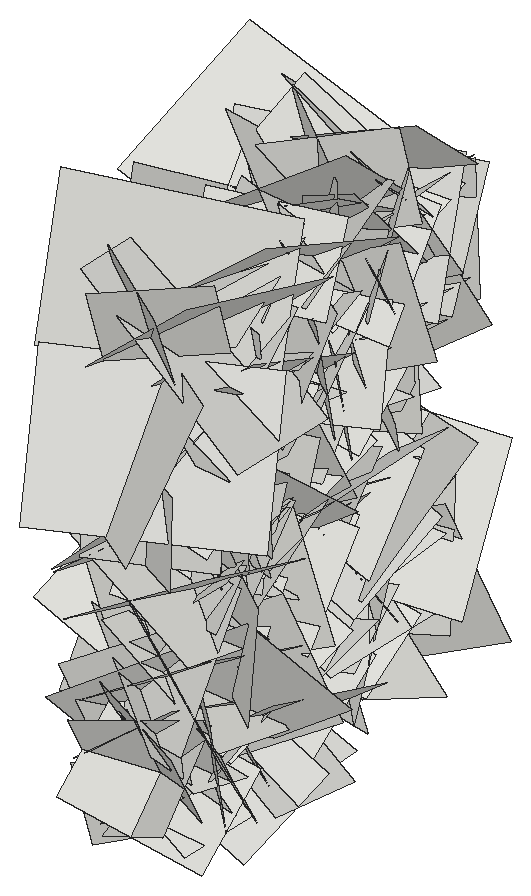
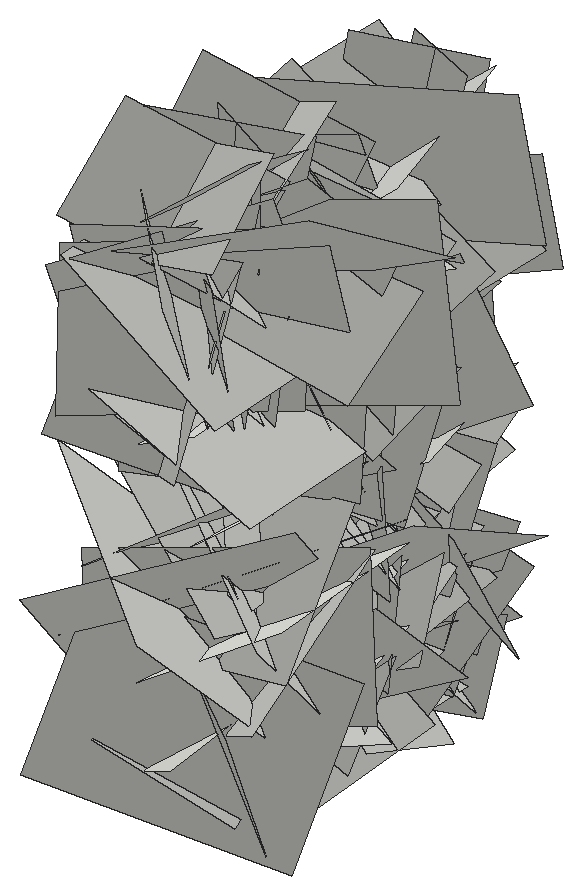
# SketchUp Ruby script. Lengths in inches.
U = 1.inch
M = Sketchup.active_model
def pt(a) = Geom::Point3d.new(a.map { |v| v * U })
def face(e, loops, mat)
  f = e.add_face(loops[0].map { |a| pt(a) })
  loops[1..].each { |l| e.add_face(l.map { |a| pt(a) }).erase! }
  f.material = f.back_material = mat if mat
  f
end
# faces: each face lists its corners as indices into pts; further lists are holes
def faces(e, pts, list, mat = nil) = list.each { |f| face(e, (f[0].is_a?(Array) ? f : [f]).map { |l| l.map { |i| pts[i] } }, mat) }
# xy, xz, yz: faces in a plane at the given z, y or x. An outline is a flat list of corners, or four numbers for a rectangle; further outlines are holes
def ring(l) = l.size == 4 ? [[l[0], l[1]], [l[2], l[1]], [l[2], l[3]], [l[0], l[3]]] : l.each_slice(2).to_a
def flat(e, list, mat, &to3) = list.each { |f| face(e, (f[0].is_a?(Array) ? f : [f]).map { |l| ring(l).map { |u, v| to3.(u, v) } }, mat) }
def xy(e, z, list, mat = nil) = flat(e, list, mat) { |x, y| [x, y, z] }
def xz(e, y, list, mat = nil) = flat(e, list, mat) { |x, z| [x, y, z] }
def yz(e, x, list, mat = nil) = flat(e, list, mat) { |y, z| [x, y, z] }
def lines(e, pts, list) = list.each { |a, b| e.add_line(pt(pts[a]), pt(pts[b])) }
# prism: a flat outline (further loops are holes) pulled along v
def prism(e, loops, v, mat = nil)
  f = face(e, loops, mat); d = Geom::Vector3d.new(v.map { |x| x * U })
  f.pushpull(f.normal.samedirection?(d) ? d.length : -d.length)
end
def box(e, o, s, mat = nil) = prism(e, [[o, [o[0] + s[0], o[1], o[2]], [o[0] + s[0], o[1] + s[1], o[2]], [o[0], o[1] + s[1], o[2]]]], [0, 0, s[2]], mat)
def at(x, y, z, deg = 0) = Geom::Transformation.translation(pt([x, y, z])) * Geom::Transformation.rotation(ORIGIN, Z_AXIS, deg.degrees)
def axes(o, x, y, z) = Geom::Transformation.new([*x, 0, *y, 0, *z, 0, *pt(o).to_a, 1])
def part(name) = M.definitions.add(name)
# library, detail: a bought-in or finely detailed component or shape, given as its bounding box
def library(name, o, s) = part(name).tap { |d| box(d.entities, o, s) }
def detail(e, o, s) = box(e.add_group.entities, o, s)
def put(e, d, t, mat = nil) = e.add_instance(d, t).tap { |i| i.material = mat if mat }
def group(e, t, mat = nil) = e.add_group.tap { |g| g.transformation = t; g.material = mat if mat }.entities
root = M.entities
c1 = part("Component\#6")
p = [[0.01,0,0],[0,3.24,4.54],[4.32,3.24,4.54],[4.33,0,0]]
faces(c1.entities,p,[[0,1,2,3]])
put(root,c1,axes([18.5,183.19,37.72],[-0.19709,-1.17807,-0.70591],[-0.26547,-0.67132,1.18631],[-1.43137,0.28672,-0.12282]))
put(root,c1,axes([18.5,179.625,37.91],[-0.28026,0.12179,-1.29213],[-0.26115,-1.29941,-0.07206],[-1.35072,0.22596,0.28204]))
put(root,c1,axes([18.5,177.28,39.83],[-0.04784,1.11638,-0.64936],[-0.22797,-0.64718,-1.09769],[-1.34988,0.06974,0.20839]))
put(root,c1,axes([18.5,183.77,26.5],[-0.0762,-1.33255,-0.21023],[-0.04546,-0.20817,1.33413],[-1.42926,0.07766,-0.03122]))
put(root,c1,axes([18.5,177.96,25.04],[-0.10915,-1.1796,-0.55067],[-0.03689,-0.5497,1.18402],[-1.37942,0.10803,0.01191]))
put(root,c1,axes([18.5,175.66,39.88],[0.03914,-0.32872,-1.22009],[-0.25418,-1.20026,0.31612],[-1.31508,0.2222,-0.09741]))
put(root,c1,axes([18.5,169.91,24.28],[0.0494,0.58776,1.07494],[-0.25393,1.05932,-0.56884],[-1.27358,-0.18841,0.15511]))
put(root,c1,axes([18.5,178.68,21.25],[-0.14964,-1.02559,0.91665],[0.24358,0.89093,1.03221],[-1.43757,0.25771,0.07948]))
put(root,c1,axes([18.5,178.09,32.9],[-0.18757,-0.47698,-1.21124],[0.23196,-1.21588,0.44684],[-1.36024,-0.14157,0.24323]))
put(root,c1,axes([18.5,178.49,34.59],[-0.00763,1.14917,-0.03145],[-0.21412,-0.03223,-1.13128],[-1.19962,-0.00155,0.20212]))
put(root,c1,axes([18.5,182.31,23.94],[0.04872,-1.30982,0.04089],[-0.01644,0.04037,1.31055],[-1.38898,-0.04642,-0.01408]))
put(root,c1,axes([18.5,174.06,31.875],[-0.08593,-0.00736,1.08266],[-0.18405,1.07173,-0.00571],[-1.1328,-0.17357,-0.0812]))
put(root,c1,axes([18.5,177.97,39.67],[0.02985,0.75948,-0.84861],[-0.27983,-0.8214,-0.74388],[-1.17429,0.21504,0.15569]))
put(root,c1,axes([18.5,180.07,24.39],[0.06666,-0.76105,0.92501],[-0.21989,0.90537,0.75899],[-1.25053,-0.19976,-0.08415]))
put(root,c1,axes([18.5,182.77,28.7],[0.0358,-0.11408,-1.31406],[0.04325,-1.31377,0.1151],[-1.39747,-0.04358,-0.0301]))
put(root,c1,axes([18.5,179.04,23.77],[-0.11323,-0.75693,-0.7774],[-0.09292,-0.77258,0.76428],[-1.14637,0.13739,0.01483]))
put(root,c1,axes([18.5,183.25,38.77],[0.07927,-0.40868,-1.12281],[-0.1988,-1.11508,0.39337],[-1.25087,0.15132,-0.13368]))
put(root,c1,axes([18.5,172.47,36.95],[-0.1233,0.89549,0.4145],[-0.21728,0.38634,-0.89217],[-1.02316,-0.18996,0.13951]))
put(root,c1,axes([18.5,175.96,26.52],[-0.03553,0.82214,0.9074],[0.07429,0.90754,-0.81968],[-1.2958,0.02948,-0.07187]))
put(root,c1,axes([18.5,182.25,27.43],[0.1955,0.46825,-1.21407],[-0.10064,-1.21809,-0.48422],[-1.37564,0.15566,-0.13711]))
put(root,c1,axes([18.5,180.75,35.09],[0.01445,0.08276,-1.11066],[-0.1396,-1.10283,-0.0838],[-1.17228,0.13235,-0.00371]))
put(root,c1,axes([14.53,172.58,29],[-0.14706,-0.68518,0.03236],[-0.10474,0.05263,0.69082],[0.71951,-0.13238,0.10718]))
put(root,c1,axes([18.5,173.84,39.64],[0.13369,1.27699,-0.41872],[0.11509,-0.42887,-1.27523],[-1.41986,0.08547,-0.14279]))
put(root,c1,axes([14.53,173.74,31.89],[-0.15856,-0.67469,0.29232],[-0.1064,0.31425,0.67394],[0.77211,-0.09525,0.1529]))
put(root,c1,axes([14.53,181.39,28.46],[-0.11732,-0.15238,-0.58962],[0.01785,-0.59981,0.15186],[0.64528,-0.01111,-0.1114]))
put(root,c1,axes([18.5,179.35,38.14],[-0.07028,1.07405,0.02302],[0.04111,0.02544,-1.07534],[-1.13802,-0.06541,-0.04027]))
put(root,c1,axes([18.5,171.47,32.36],[-0.16942,0.96147,-0.31887],[0.08969,-0.30901,-0.97416],[-1.06999,-0.17814,-0.03117]))
put(root,c1,axes([18.5,172.46,21.25],[-0.14489,-0.73421,0.72244],[0.08794,0.71856,0.74596],[-1.0883,0.15581,-0.0359]))
put(root,c1,axes([14.53,180.42,25.12],[-0.17902,-0.88337,-0.09354],[-0.21931,-0.05348,0.8786],[0.91571,-0.1855,0.19214]))
put(root,c1,axes([14.53,176.07,37.03],[-0.15674,-0.62528,-0.09698],[0.10666,-0.12156,0.63036],[0.66219,-0.12843,-0.12449]))
put(root,c1,axes([18.5,171.95,33.74],[0.07102,0.70639,0.8167],[-0.11892,0.8184,-0.69866],[-1.13841,-0.04142,0.12393]))
put(root,c1,axes([14.53,178.13,40.15],[-0.04908,0.64392,0.19174],[-0.08573,0.18545,-0.64234],[0.70699,0.06719,-0.06458]))
put(root,c1,axes([18.5,178.01,21.81],[-0.00864,0.40014,0.99077],[0.02339,0.99065,-0.39991],[-1.13239,0.01741,-0.01582]))
put(root,c1,axes([14.53,170.73,19.61],[-0.06378,-0.15247,0.68566],[-0.07422,0.68605,0.14641],[0.74085,0.05561,0.0737]))
put(root,c1,axes([14.53,180.68,27.18],[-0.06604,-0.60003,0.10008],[0.10227,0.08959,0.59716],[0.63666,-0.07663,-0.08554]))
put(root,c1,axes([18.5,174.78,20.26],[-0.10048,-0.39109,0.79293],[-0.10042,0.79738,0.38196],[-0.93179,-0.04376,-0.12667]))
put(root,c1,axes([18.5,173.31,35.98],[0.01252,1.07454,-0.37217],[0.12805,-0.37127,-1.06811],[-1.19858,-0.02844,-0.11799]))
put(root,c1,axes([18.5,183.67,38.38],[-0.04708,0.10578,-1.15378],[0.2342,-1.13267,-0.11235],[-1.2056,-0.22416,0.02323]))
put(root,c1,axes([14.53,176.44,21.6],[-0.04345,0.60879,-0.00304],[0.10651,0.00376,-0.60183],[0.63647,0.04093,0.10051]))
put(root,c1,axes([14.53,178.15,33.23],[0.08938,-0.00525,-0.60269],[-0.06829,-0.60515,-0.00374],[0.63521,-0.06432,0.0844]))
put(root,c1,axes([14.53,173.11,21.9],[-0.05319,-0.68826,0.19248],[-0.04456,0.19546,0.68797],[0.75624,-0.03689,0.05408]))
put(root,c1,axes([18.5,174.9,23.69],[0.06803,0.90477,0.33383],[-0.16872,0.33992,-0.89067],[-1.00823,0.00417,0.17157]))
put(root,c1,axes([14.53,182.27,37.76],[-0.22679,0.05489,-0.89691],[-0.06736,-0.9206,-0.04118],[0.95012,-0.05216,-0.217]))
put(root,c1,axes([18.5,176.05,33.17],[-0.01986,0.50916,-0.88553],[0.06176,-0.8837,-0.50934],[-1.08099,-0.05984,-0.01283]))
put(root,c1,axes([18.5,182.77,28.15],[0.11013,-1.0722,-0.31704],[0.03816,-0.31503,1.07721],[-1.18456,-0.10983,0.00522]))
put(root,c1,axes([18.5,185.38,28.27],[0.28552,-0.8956,-0.93898],[0.07116,-0.9481,0.92355],[-1.37362,-0.23528,-0.14733]))
put(root,c1,axes([14.53,175.43,34.87],[-0.0411,0.62613,0.35799],[-0.03637,0.3565,-0.62724],[0.76365,0.05068,-0.01061]))
put(root,c1,axes([14.53,173.67,32.24],[-0.05341,-0.65994,-0.37026],[-0.06447,-0.36634,0.66124],[0.79951,-0.07362,0.02859]))
put(root,c1,axes([18.5,174.01,26.46],[0.07872,-0.97306,0.24072],[-0.0738,0.23579,0.97461],[-1.05998,-0.08868,-0.04998]))
put(root,c1,axes([18.5,170.16,39.2],[0.24703,1.2789,-0.21613],[0.13589,-0.24123,-1.28918],[-1.36812,0.20696,-0.16707]))
put(root,c1,axes([14.53,173.15,22.23],[0.01199,-0.5915,0.12784],[0.10227,0.12799,0.58366],[0.63327,-0.00947,-0.09668]))
put(root,c1,axes([18.5,167.34,31.77],[0.2501,0.51374,1.1242],[0.05799,1.13903,-0.532],[-1.3089,0.14863,0.19123]))
put(root,c1,axes([14.53,174.375,32.02],[-0.18574,0.64681,-0.5499],[-0.00393,-0.56207,-0.65994],[0.8999,0.13105,-0.11638]))
put(root,c1,axes([14.53,171.42,39.46],[0.01769,0.21401,-0.61924],[0.03571,-0.6189,-0.21298],[0.69357,0.02641,0.02676]))
put(root,c1,axes([14.53,180.11,41],[-0.0874,0.13713,-0.78202],[-0.02965,-0.78624,-0.13492],[0.84107,-0.01347,-0.08602]))
put(root,c1,axes([18.5,182.1,27.04],[0.18817,-1.1788,-0.21223],[0.10509,-0.19936,1.19019],[-1.26526,-0.19187,0.06729]))
put(root,c1,axes([18.5,177.13,31.79],[0.078,-0.30439,1.03044],[0.07955,1.03178,0.29943],[-1.13614,0.05135,0.09171]))
put(root,c1,axes([18.5,172.13,35.78],[-0.07615,0.65901,-0.5201],[-0.04859,-0.52431,-0.658],[-0.88857,-0.02781,0.08055]))
put(root,c1,axes([18.5,172.625,27.43],[0.01975,0.58315,0.74345],[-0.01761,0.74368,-0.58292],[-1.00141,-0.00157,0.02491]))
put(root,c1,axes([18.5,173.5,20.5],[0.29119,-0.77592,0.90535],[-0.00734,0.92801,0.79744],[-1.26387,-0.18415,0.20396]))
put(root,c1,axes([18.5,181.8125,37.17],[0.0246,-0.63961,0.56311],[-0.17949,0.54862,0.63013],[-0.88529,-0.129,-0.11211]))
put(root,c1,axes([14.53,177.7,39.03],[-0.08239,-0.33737,-0.64844],[0.10668,-0.65083,0.32654],[0.76743,0.05425,-0.11501]))
put(root,c1,axes([18.5,176.41,32.2],[-0.11408,-0.0942,-0.79779],[-0.0272,-0.8041,0.09841],[-0.85109,0.03832,0.10379]))
put(root,c1,axes([18.5,171.36,22.89],[-0.02535,0.88672,0.32576],[0.06435,0.32663,-0.88464],[-0.99927,-0.00146,-0.06523]))
put(root,c1,axes([18.5,178.05,19.9375],[0.14578,-1.0409,0.22357],[0.02192,0.228,1.04879],[-1.1283,-0.13006,0.04926]))
put(root,c1,axes([18.5,180.04,24.28],[-0.15161,0.71603,-0.23582],[-0.04269,-0.24694,-0.72538],[-0.79796,-0.12284,0.08362]))
put(root,c1,axes([14.53,173.29,20.87],[0.09428,-0.62013,-0.08152],[0.03551,-0.0775,0.6261],[0.66205,0.09247,-0.02197]))
put(root,c1,axes([14.53,173.36,27.66],[-0.12062,0.63946,0.63128],[-0.06443,0.62939,-0.6485],[0.9503,0.12384,0.03616]))
put(root,c1,axes([18.5,175.14,30.45],[0.22771,0.17317,-1.07869],[-0.0194,-1.09862,-0.18001],[-1.15789,0.05246,-0.20912]))
put(root,c1,axes([18.5,184.3,37.98],[0.01849,-0.42221,-1.00939],[0.24573,-0.98518,0.41609],[-1.13346,-0.22047,0.07374]))
put(root,c1,axes([14.53,172.01,32.68],[0.01531,-0.04852,-0.71126],[0.05574,-0.70939,0.04946],[0.75363,0.05345,0.01079]))
put(root,c1,axes([18.5,172,20.82],[0.19013,-0.4174,1.11707],[0.18593,1.12659,0.39279],[-1.25031,0.10406,0.22828]))
put(root,c1,axes([18.5,178.01,36.42],[-0.04909,-0.68925,0.58112],[0.09024,0.57594,0.68989],[-0.95135,0.0902,0.03545]))
put(root,c1,axes([18.5,174.95,31.63],[-0.12097,-0.07785,-0.70642],[-0.09105,-0.70871,0.09198],[-0.74781,0.09888,0.10307]))
put(root,c1,axes([14.53,171.52,27.71],[-0.03995,0.48298,0.66079],[-0.01207,0.66111,-0.48387],[0.8675,0.03144,0.0237]))
put(root,c1,axes([18.5,174.16,29.86],[-0.19319,0.59277,-0.26834],[-0.07097,-0.29428,-0.60458],[-0.68606,-0.13648,0.1381]))
put(root,c1,axes([18.5,171.18,26.98],[0.09963,0.88743,-0.23237],[-0.05305,-0.22828,-0.89204],[-0.97094,0.10354,0.02489]))
put(root,c1,axes([18.5,169.05,21.98],[-0.04882,0.58162,0.59704],[0.02934,0.59868,-0.58109],[-0.88303,-0.01226,-0.05232]))
put(root,c1,axes([18.5,176.26,32.94],[-0.03084,0.60524,0.59943],[0.03406,0.60013,-0.60439],[-0.90231,0.00196,-0.0433]))
put(root,c1,axes([18.5,174.875,32.24],[-0.12053,0.70886,0.38052],[0.08644,0.39248,-0.70676],[-0.84842,-0.06072,-0.12606]))
put(root,c1,axes([18.5,177.89,30.77],[-0.05678,-0.11721,0.8526],[0.09083,0.84928,0.12214],[-0.90772,0.09231,-0.04111]))
put(root,c1,axes([18.5,177.99,23.55],[-0.04107,0.5427,0.4395],[-0.20397,0.41484,-0.52921],[-0.71159,-0.15024,0.12632]))
put(root,c1,axes([18.5,174.67,32.54],[0.17055,0.3665,0.95024],[0.03456,0.95968,-0.37566],[-1.07902,0.08867,0.13816]))
put(root,c1,axes([18.5,176.52,27.27],[-0.06139,-0.83333,-0.30669],[0.14477,-0.31205,0.82208],[-0.93005,0.00643,0.1482]))
put(root,c1,axes([14.53,180.66,33.34],[-0.08177,-0.45253,0.73357],[0.03972,0.73405,0.45677],[0.91278,-0.07248,0.04584]))
put(root,c1,axes([14.53,181.67,36.78],[-0.05967,0.56874,-0.94691],[-0.29528,-0.9248,-0.5389],[1.13301,-0.21107,-0.19031]))
put(root,c1,axes([14.53,170.91,25.11],[0.00896,0.33986,-0.6335],[0.15678,-0.62081,-0.33108],[0.74574,0.12644,0.07722]))
put(root,c1,axes([18.5,182.09,31.375],[-0.0562,-0.72005,0.10613],[-0.07977,0.11126,0.71729],[-0.76737,0.04117,-0.08234]))
put(root,c1,axes([14.53,175.72,36.8],[-0.15665,0.75943,0.7145],[-0.11122,0.70715,-0.77331],[1.09966,0.17971,0.02357]))
put(root,c1,axes([18.5,175.72,36.8],[0.15665,0.75943,0.7145],[0.11122,0.70715,-0.77331],[-1.09966,0.17971,0.02357]))
put(root,c1,axes([14.53,182.09,31.375],[0.0562,-0.72005,0.10613],[0.07977,0.11126,0.71729],[0.76737,0.04117,-0.08234]))
put(root,c1,axes([18.5,170.91,25.11],[-0.00896,0.33986,-0.6335],[-0.15678,-0.62081,-0.33108],[-0.74574,0.12644,0.07722]))
put(root,c1,axes([18.5,181.67,36.78],[0.05967,0.56874,-0.94691],[0.29528,-0.9248,-0.5389],[-1.13301,-0.21107,-0.19031]))
put(root,c1,axes([18.5,180.66,33.34],[0.08177,-0.45253,0.73357],[-0.03972,0.73405,0.45677],[-0.91278,-0.07248,0.04584]))
put(root,c1,axes([14.53,176.52,27.27],[0.06139,-0.83333,-0.30669],[-0.14477,-0.31205,0.82208],[0.93005,0.00643,0.1482]))
put(root,c1,axes([14.53,174.67,32.54],[-0.17055,0.3665,0.95024],[-0.03456,0.95968,-0.37566],[1.07902,0.08867,0.13816]))
put(root,c1,axes([14.53,177.99,23.55],[0.04107,0.5427,0.4395],[0.20397,0.41484,-0.52921],[0.71159,-0.15024,0.12632]))
put(root,c1,axes([14.53,177.89,30.77],[0.05678,-0.11721,0.8526],[-0.09083,0.84928,0.12214],[0.90772,0.09231,-0.04111]))
put(root,c1,axes([14.53,174.875,32.24],[0.12053,0.70886,0.38052],[-0.08644,0.39248,-0.70676],[0.84842,-0.06072,-0.12606]))
put(root,c1,axes([14.53,176.26,32.94],[0.03084,0.60524,0.59943],[-0.03406,0.60013,-0.60439],[0.90231,0.00196,-0.0433]))
put(root,c1,axes([14.53,169.05,21.98],[0.04882,0.58162,0.59704],[-0.02934,0.59868,-0.58109],[0.88303,-0.01226,-0.05232]))
put(root,c1,axes([14.53,171.18,26.98],[-0.09963,0.88743,-0.23237],[0.05305,-0.22828,-0.89204],[0.97094,0.10354,0.02489]))
put(root,c1,axes([14.53,174.16,29.86],[0.19319,0.59277,-0.26834],[0.07097,-0.29428,-0.60458],[0.68606,-0.13648,0.1381]))
put(root,c1,axes([18.5,171.52,27.71],[0.03995,0.48298,0.66079],[0.01207,0.66111,-0.48387],[-0.8675,0.03144,0.0237]))
put(root,c1,axes([14.53,174.95,31.63],[0.12097,-0.07785,-0.70642],[0.09105,-0.70871,0.09198],[0.74781,0.09888,0.10307]))
put(root,c1,axes([14.53,178.01,36.42],[0.04909,-0.68925,0.58112],[-0.09024,0.57594,0.68989],[0.95135,0.0902,0.03545]))
put(root,c1,axes([14.53,172,20.82],[-0.19013,-0.4174,1.11707],[-0.18593,1.12659,0.39279],[1.25031,0.10406,0.22828]))
put(root,c1,axes([18.5,172.01,32.68],[-0.01531,-0.04852,-0.71126],[-0.05574,-0.70939,0.04946],[-0.75363,0.05345,0.01079]))
put(root,c1,axes([14.53,184.3,37.98],[-0.01849,-0.42221,-1.00939],[-0.24573,-0.98518,0.41609],[1.13346,-0.22047,0.07374]))
put(root,c1,axes([14.53,175.14,30.45],[-0.22771,0.17317,-1.07869],[0.0194,-1.09862,-0.18001],[1.15789,0.05246,-0.20912]))
put(root,c1,axes([18.5,173.36,27.66],[0.12062,0.63946,0.63128],[0.06443,0.62939,-0.6485],[-0.9503,0.12384,0.03616]))
put(root,c1,axes([18.5,173.29,20.87],[-0.09428,-0.62013,-0.08152],[-0.03551,-0.0775,0.6261],[-0.66205,0.09247,-0.02197]))
put(root,c1,axes([14.53,180.04,24.28],[0.15161,0.71603,-0.23582],[0.04269,-0.24694,-0.72538],[0.79796,-0.12284,0.08362]))
put(root,c1,axes([14.53,178.05,19.9375],[-0.14578,-1.0409,0.22357],[-0.02192,0.228,1.04879],[1.1283,-0.13006,0.04926]))
put(root,c1,axes([14.53,171.36,22.89],[0.02535,0.88672,0.32576],[-0.06435,0.32663,-0.88464],[0.99927,-0.00146,-0.06523]))
put(root,c1,axes([14.53,176.41,32.2],[0.11408,-0.0942,-0.79779],[0.0272,-0.8041,0.09841],[0.85109,0.03832,0.10379]))
put(root,c1,axes([18.5,177.7,39.03],[0.08239,-0.33737,-0.64844],[-0.10668,-0.65083,0.32654],[-0.76743,0.05425,-0.11501]))
put(root,c1,axes([14.53,181.8125,37.17],[-0.0246,-0.63961,0.56311],[0.17949,0.54862,0.63013],[0.88529,-0.129,-0.11211]))
put(root,c1,axes([14.53,173.5,20.5],[-0.29119,-0.77592,0.90535],[0.00734,0.92801,0.79744],[1.26387,-0.18415,0.20396]))
put(root,c1,axes([14.53,172.625,27.43],[-0.01975,0.58315,0.74345],[0.01761,0.74368,-0.58292],[1.00141,-0.00157,0.02491]))
put(root,c1,axes([14.53,172.13,35.78],[0.07615,0.65901,-0.5201],[0.04859,-0.52431,-0.658],[0.88857,-0.02781,0.08055]))
put(root,c1,axes([14.53,177.13,31.79],[-0.078,-0.30439,1.03044],[-0.07955,1.03178,0.29943],[1.13614,0.05135,0.09171]))
put(root,c1,axes([14.53,182.1,27.04],[-0.18817,-1.1788,-0.21223],[-0.10509,-0.19936,1.19019],[1.26526,-0.19187,0.06729]))
put(root,c1,axes([18.5,180.11,41],[0.0874,0.13713,-0.78202],[0.02965,-0.78624,-0.13492],[-0.84107,-0.01347,-0.08602]))
put(root,c1,axes([18.5,171.42,39.46],[-0.01769,0.21401,-0.61924],[-0.03571,-0.6189,-0.21298],[-0.69357,0.02641,0.02676]))
put(root,c1,axes([18.5,174.375,32.02],[0.18574,0.64681,-0.5499],[0.00393,-0.56207,-0.65994],[-0.8999,0.13105,-0.11638]))
put(root,c1,axes([14.53,167.34,31.77],[-0.2501,0.51374,1.1242],[-0.05799,1.13903,-0.532],[1.3089,0.14863,0.19123]))
put(root,c1,axes([18.5,173.15,22.23],[-0.01199,-0.5915,0.12784],[-0.10227,0.12799,0.58366],[-0.63327,-0.00947,-0.09668]))
put(root,c1,axes([14.53,170.16,39.2],[-0.24703,1.2789,-0.21613],[-0.13589,-0.24123,-1.28918],[1.36812,0.20696,-0.16707]))
put(root,c1,axes([14.53,174.01,26.46],[-0.07872,-0.97306,0.24072],[0.0738,0.23579,0.97461],[1.05998,-0.08868,-0.04998]))
put(root,c1,axes([18.5,173.67,32.24],[0.05341,-0.65994,-0.37026],[0.06447,-0.36634,0.66124],[-0.79951,-0.07362,0.02859]))
put(root,c1,axes([18.5,175.43,34.87],[0.0411,0.62613,0.35799],[0.03637,0.3565,-0.62724],[-0.76365,0.05068,-0.01061]))
put(root,c1,axes([14.53,185.38,28.27],[-0.28552,-0.8956,-0.93898],[-0.07116,-0.9481,0.92355],[1.37362,-0.23528,-0.14733]))
